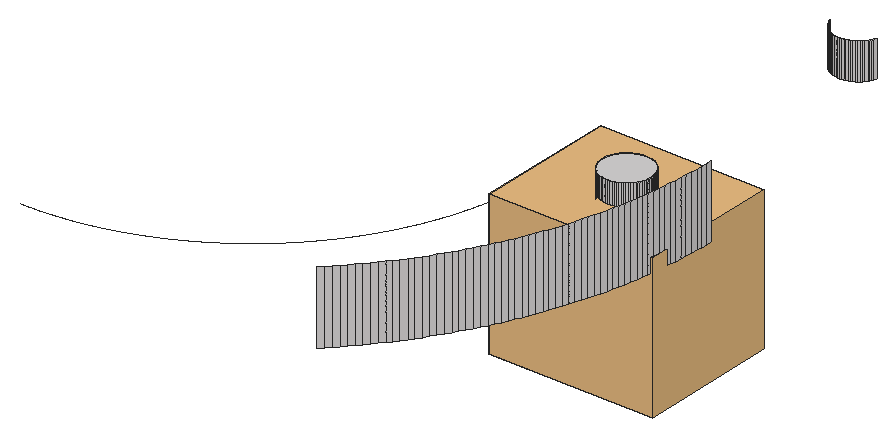
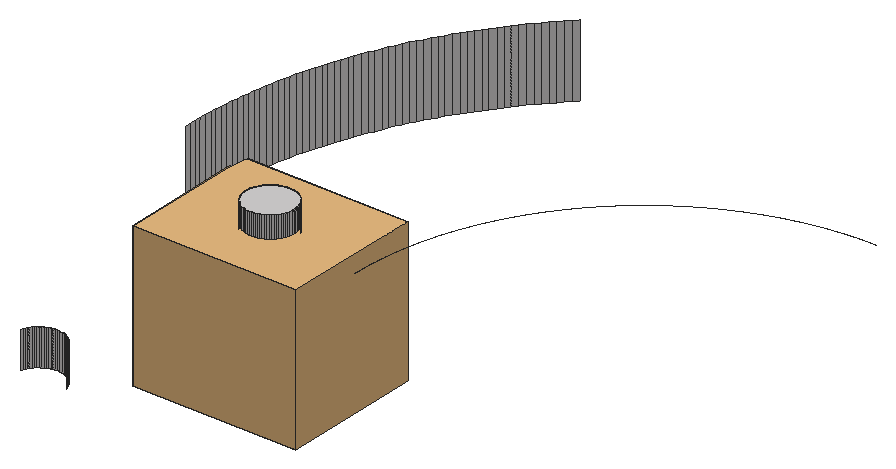
# SketchUp Ruby script. Lengths in inches.
U = 1.inch
M = Sketchup.active_model
def pt(a) = Geom::Point3d.new(a.map { |v| v * U })
def face(e, loops, mat)
  f = e.add_face(loops[0].map { |a| pt(a) })
  loops[1..].each { |l| e.add_face(l.map { |a| pt(a) }).erase! }
  f.material = f.back_material = mat if mat
  f
end
# faces: each face lists its corners as indices into pts; further lists are holes
def faces(e, pts, list, mat = nil) = list.each { |f| face(e, (f[0].is_a?(Array) ? f : [f]).map { |l| l.map { |i| pts[i] } }, mat) }
# xy, xz, yz: faces in a plane at the given z, y or x. An outline is a flat list of corners, or four numbers for a rectangle; further outlines are holes
def ring(l) = l.size == 4 ? [[l[0], l[1]], [l[2], l[1]], [l[2], l[3]], [l[0], l[3]]] : l.each_slice(2).to_a
def flat(e, list, mat, &to3) = list.each { |f| face(e, (f[0].is_a?(Array) ? f : [f]).map { |l| ring(l).map { |u, v| to3.(u, v) } }, mat) }
def xy(e, z, list, mat = nil) = flat(e, list, mat) { |x, y| [x, y, z] }
def xz(e, y, list, mat = nil) = flat(e, list, mat) { |x, z| [x, y, z] }
def yz(e, x, list, mat = nil) = flat(e, list, mat) { |y, z| [x, y, z] }
def lines(e, pts, list) = list.each { |a, b| e.add_line(pt(pts[a]), pt(pts[b])) }
# prism: a flat outline (further loops are holes) pulled along v
def prism(e, loops, v, mat = nil)
  f = face(e, loops, mat); d = Geom::Vector3d.new(v.map { |x| x * U })
  f.pushpull(f.normal.samedirection?(d) ? d.length : -d.length)
end
def box(e, o, s, mat = nil) = prism(e, [[o, [o[0] + s[0], o[1], o[2]], [o[0] + s[0], o[1] + s[1], o[2]], [o[0], o[1] + s[1], o[2]]]], [0, 0, s[2]], mat)
def at(x, y, z, deg = 0) = Geom::Transformation.translation(pt([x, y, z])) * Geom::Transformation.rotation(ORIGIN, Z_AXIS, deg.degrees)
def axes(o, x, y, z) = Geom::Transformation.new([*x, 0, *y, 0, *z, 0, *pt(o).to_a, 1])
def part(name) = M.definitions.add(name)
# library, detail: a bought-in or finely detailed component or shape, given as its bounding box
def library(name, o, s) = part(name).tap { |d| box(d.entities, o, s) }
def detail(e, o, s) = box(e.add_group.entities, o, s)
def put(e, d, t, mat = nil) = e.add_instance(d, t).tap { |i| i.material = mat if mat }
def group(e, t, mat = nil) = e.add_group.tap { |g| g.transformation = t; g.material = mat if mat }.entities
root = M.entities
M.materials.add("[Quartz Light Brown]").color = [215, 212, 212]
c1 = library("3",[-5.26,-4.28,-11.86],[13.52,11.56,11.86])
xy(root,483,[[494.91,318.7,494.59,318.74,494.44,318.78,494.29,318.83,494.15,318.89,494.01,318.96,493.875,319.05,493.75,319.14,493.63,319.24,493.52,319.36,493.42,319.48,493.33,319.6,493.25,319.74,493.18,319.88,493.12,320.02,493.07,320.17,493.04,320.33,493.01,320.48,493,320.64,493,320.8,493.02,320.95,493.04,321.11,493.08,321.26,493.13,321.41,493.19,321.55,493.26,321.69,493.35,321.83,493.44,321.95,493.54,322.07,493.65,322.18,493.77,322.28,493.9,322.37,494.04,322.45,494.18,322.52,494.32,322.58,494.47,322.63,494.625,322.67,494.78,322.6875,494.9375,322.7,495.09,322.7,495.25,322.69,495.41,322.66,495.56,322.62,495.71,322.57,495.85,322.51,495.99,322.4375,496.125,322.35,496.25,322.26,496.37,322.16,496.48,322.05,496.58,321.93,496.67,321.8,496.75,321.66,496.82,321.52,496.88,321.38,496.93,321.23,496.96,321.08,496.99,320.92,497,320.76,497,320.61,496.96,320.29,496.92,320.14,496.87,319.99,496.81,319.85,496.74,319.71,496.56,319.45,496.46,319.33,496.35,319.22,496.23,319.12,496.1,319.03,495.96,318.95,495.82,318.88,495.68,318.82,495.53,318.77,495.22,318.71,495.0625,318.7]],"[Quartz Light Brown]")
xz(root,318.7,[[494.91,480,495.0625,483]],"[Quartz Light Brown]")
xz(root,322.7,[[494.9375,480,495.09,483]],"[Quartz Light Brown]")
xz(root,342.7,[[494.91,480,495.0625,483]],"[Quartz Light Brown]")
yz(root,493,[[320.64,480,320.8,483]],"[Quartz Light Brown]")
yz(root,497,[[320.61,480,320.76,483]],"[Quartz Light Brown]")
yz(root,502,[[320.2,480,320.7,486]],"[Quartz Light Brown]")
p = [[490.87,293.83,480],[491.22,294.18,480],[491.22,294.18,486],[490.87,293.83,486],[491.5625,294.54,480],[491.5625,294.54,486],
  [491.9,294.91,480],[491.9,294.91,486],[492.24,295.27,480],[492.24,295.27,486],[492.57,295.65,480],[492.57,295.65,486],
  [492.9,296.02,480],[492.9,296.02,486],[493.22,296.4,480],[493.22,296.4,486],[493.53,296.79,480],[493.53,296.79,486],
  [493.84,297.18,480],[493.84,297.18,486],[494.15,297.57,480],[494.15,297.57,486],[494.45,297.96,480],[494.45,297.96,486],
  [494.74,298.37,480],[494.74,298.37,486],[495.03,298.77,480],[495.03,298.77,486],[495.32,299.18,480],[495.32,299.18,486],
  [495.6,299.59,480],[495.6,299.59,486],[495.87,300,480],[495.87,300,486],[496.14,300.42,480],[496.14,300.42,486],
  [496.4,300.85,480],[496.4,300.85,486],[496.66,301.27,480],[496.66,301.27,486],[496.91,301.7,480],[496.91,301.7,486],
  [497.15,302.13,480],[497.15,302.13,486],[497.4,302.57,480],[497.4,302.57,486],[497.63,303.01,480],[497.63,303.01,486],
  [497.86,303.45,480],[497.86,303.45,486],[498.08,303.89,480],[498.08,303.89,486],[498.3,304.34,480],[498.3,304.34,486],
  [498.51,304.79,480],[498.51,304.79,486],[498.71,305.25,480],[498.71,305.25,486],[498.91,305.7,480],[498.91,305.7,486],
  [499.11,306.16,480],[499.11,306.16,486],[499.29,306.62,480],[499.29,306.62,486],[499.48,307.08,480],[499.48,307.08,486],
  [499.65,307.55,480],[499.65,307.55,486],[499.82,308.02,480],[499.82,308.02,486],[499.98,308.49,480],[499.98,308.49,486],
  [500.14,308.96,480],[500.14,308.96,486],[500.29,309.43,480],[500.29,309.43,486],[500.44,309.91,480],[500.44,309.91,486],
  [500.57,310.39,480],[500.57,310.39,486],[500.71,310.87,480],[500.71,310.87,486],[500.83,311.35,480],[500.83,311.35,486],
  [500.95,311.83,480],[500.95,311.83,486],[501.0625,312.31,480],[501.0625,312.31,486],[501.17,312.8,480],[501.17,312.8,486],
  [501.27,313.29,480],[501.27,313.29,486],[501.36,313.78,480],[501.36,313.78,486],[501.45,314.27,480],[501.45,314.27,486],
  [501.53,314.76,480],[501.53,314.76,486],[501.61,315.25,480],[501.61,315.25,486],[501.67,315.74,480],[501.67,315.74,486],
  [501.74,316.23,480],[501.74,316.23,486],[501.79,316.73,480],[501.79,316.73,486],[501.84,317.22,480],[501.84,317.22,486],
  [501.88,317.72,480],[501.88,317.72,486],[501.92,318.22,480],[501.92,318.22,486],[501.95,318.71,480],[501.95,318.71,486],
  [494.59,318.74,480],[494.44,318.78,480],[494.44,318.78,483],[494.59,318.74,483],[494.75,318.72,480],[494.75,318.72,483],
  [494.91,318.7,480],[494.91,318.7,483],[495.22,318.71,480],[495.0625,318.7,480],[495.0625,318.7,483],[495.22,318.71,483],
  [495.375,318.74,480],[495.375,318.74,483],[495.53,318.77,480],[495.53,318.77,483],[501.97,319.21,480],[501.97,319.21,486],
  [494.29,318.83,480],[494.15,318.89,480],[494.15,318.89,483],[494.29,318.83,483],[495.68,318.82,480],[495.68,318.82,483],
  [495.82,318.88,480],[495.82,318.88,483],[494.01,318.96,480],[494.01,318.96,483],[495.96,318.95,480],[495.96,318.95,483],
  [496.1,319.03,480],[496.1,319.03,483],[493.875,319.05,480],[493.75,319.14,480],[493.75,319.14,483],[493.875,319.05,483],
  [496.23,319.12,480],[496.23,319.12,483],[493.63,319.24,480],[493.63,319.24,483],[496.35,319.22,480],[496.35,319.22,483],
  [493.52,319.36,480],[493.52,319.36,483],[496.46,319.33,480],[496.46,319.33,483],[501.99,319.71,480],[501.99,319.71,486],
  [496.56,319.45,480],[496.56,319.45,483],[493.42,319.48,480],[493.42,319.48,483],[493.33,319.6,480],[493.33,319.6,483],
  [496.65,319.58,480],[496.65,319.58,483],[493.25,319.74,480],[493.25,319.74,483],[496.74,319.71,480],[496.74,319.71,483],
  [493.18,319.88,480],[493.18,319.88,483],[496.81,319.85,480],[496.81,319.85,483],[502,320.2,480],[502,320.2,486],
  [496.87,319.99,480],[496.87,319.99,483],[493.12,320.02,480],[493.12,320.02,483],[493.07,320.17,480],[493.07,320.17,483],
  [496.92,320.14,480],[496.92,320.14,483],[496.96,320.29,480],[496.96,320.29,483],[493.04,320.33,480],[493.04,320.33,483],
  [493.01,320.48,480],[493.01,320.48,483],[496.98,320.45,480],[496.98,320.45,483],[497,320.61,480],[497,320.61,483],
  [493,320.64,480],[493,320.64,483],[493,320.8,480],[493.02,320.95,480],[493.02,320.95,483],[493,320.8,483],
  [496.99,320.92,480],[497,320.76,480],[497,320.76,483],[496.99,320.92,483],[496.96,321.08,480],[496.96,321.08,483],
  [493.04,321.11,480],[493.04,321.11,483],[493.08,321.26,480],[493.08,321.26,483],[496.93,321.23,480],[496.93,321.23,483],
  [496.88,321.38,480],[496.88,321.38,483],[493.13,321.41,480],[493.13,321.41,483],[493.19,321.55,480],[493.19,321.55,483],
  [496.82,321.52,480],[496.82,321.52,483],[496.75,321.66,480],[496.75,321.66,483],[493.26,321.69,480],[493.26,321.69,483],
  [493.35,321.83,480],[493.35,321.83,483],[496.67,321.8,480],[496.67,321.8,483],[493.44,321.95,480],[493.44,321.95,483],
  [496.58,321.93,480],[496.58,321.93,483],[496.48,322.05,480],[496.48,322.05,483],[493.54,322.07,480],[493.54,322.07,483],
  [496.37,322.16,480],[496.37,322.16,483],[493.65,322.18,480],[493.65,322.18,483],[493.77,322.28,480],[493.77,322.28,483],
  [496.25,322.26,480],[496.25,322.26,483],[493.9,322.37,480],[493.9,322.37,483],[496.125,322.35,480],[496.125,322.35,483],
  [494.04,322.45,480],[494.04,322.45,483],[495.85,322.51,480],[495.99,322.4375,480],[495.99,322.4375,483],[495.85,322.51,483],
  [494.18,322.52,480],[494.18,322.52,483],[494.32,322.58,480],[494.32,322.58,483],[495.71,322.57,480],[495.71,322.57,483],
  [494.47,322.63,480],[494.47,322.63,483],[494.625,322.67,480],[494.625,322.67,483],[495.41,322.66,480],[495.56,322.62,480],
  [495.56,322.62,483],[495.41,322.66,483],[494.78,322.6875,480],[494.78,322.6875,483],[494.9375,322.7,480],[494.9375,322.7,483],
  [495.09,322.7,480],[495.25,322.69,480],[495.25,322.69,483],[495.09,322.7,483],[494.59,342.74,480],[494.44,342.78,480],
  [494.44,342.78,483],[494.59,342.74,483],[494.75,342.72,480],[494.75,342.72,483],[494.91,342.7,480],[494.91,342.7,483],
  [495.22,342.71,480],[495.0625,342.7,480],[495.0625,342.7,483],[495.22,342.71,483],[495.375,342.74,480],[495.375,342.74,483],
  [495.53,342.77,480],[495.53,342.77,483],[494.29,342.83,480],[494.15,342.89,480],[494.15,342.89,483],[494.29,342.83,483],
  [495.68,342.82,480],[495.68,342.82,483],[495.82,342.88,480],[495.82,342.88,483],[494.01,342.96,480],[494.01,342.96,483],
  [495.96,342.95,480],[495.96,342.95,483],[496.1,343.03,480],[496.1,343.03,483],[493.875,343.05,480],[493.75,343.14,480],
  [493.75,343.14,483],[493.875,343.05,483],[496.23,343.12,480],[496.23,343.12,483],[493.63,343.24,480],[493.63,343.24,483],
  [496.35,343.22,480],[496.35,343.22,483],[493.52,343.36,480],[493.52,343.36,483],[496.46,343.33,480],[496.46,343.33,483],
  [496.56,343.45,480],[496.56,343.45,483],[493.42,343.48,480],[493.42,343.48,483],[493.33,343.6,480],[493.33,343.6,483],
  [496.65,343.58,480],[496.65,343.58,483],[493.25,343.74,480],[493.25,343.74,483],[496.74,343.71,480],[496.74,343.71,483],
  [493.18,343.88,480],[493.18,343.88,483],[496.81,343.85,480],[496.81,343.85,483],[496.87,343.99,480],[496.87,343.99,483],
  [493.12,344.02,480],[493.12,344.02,483],[493.07,344.17,480],[493.07,344.17,483],[496.92,344.14,480],[496.92,344.14,483],
  [464,296.7,480],[464.3125,296.7,480],[464.63,296.71,480],[464.94,296.72,480],[465.26,296.73,480],[465.57,296.75,480],
  [465.88,296.77,480],[466.2,296.8,480],[466.51,296.83,480],[466.82,296.87,480],[467.13,296.91,480],[467.44,296.95,480],
  [467.75,297,480],[468.0625,297.05,480],[468.375,297.1,480],[468.68,297.16,480],[468.99,297.23,480],[469.3,297.29,480],
  [469.6,297.36,480],[469.91,297.4375,480],[470.21,297.52,480],[470.51,297.6,480],[470.82,297.6875,480],[471.12,297.78,480],
  [471.42,297.875,480],[471.71,297.97,480],[472.01,298.08,480],[472.31,298.18,480],[472.6,298.3,480],[472.89,298.41,480],
  [473.18,298.53,480],[473.47,298.65,480],[473.76,298.78,480],[474.05,298.91,480],[474.33,299.04,480],[474.61,299.18,480],
  [474.9,299.32,480],[475.17,299.46,480],[475.45,299.61,480],[475.73,299.76,480],[476,299.92,480],[476.27,300.08,480],
  [476.54,300.24,480],[476.81,300.4,480],[477.07,300.57,480],[477.33,300.75,480],[477.59,300.92,480],[477.85,301.1,480],
  [478.11,301.28,480],[478.36,301.47,480],[478.61,301.66,480],[478.86,301.85,480],[479.1,302.05,480],[479.35,302.25,480],
  [479.59,302.45,480],[479.82,302.66,480],[480.06,302.87,480],[480.29,303.08,480],[480.52,303.29,480],[480.75,303.51,480],
  [480.97,303.73,480],[481.19,303.95,480],[481.41,304.18,480],[481.625,304.41,480],[481.84,304.64,480],[482.04,304.875,480],
  [482.25,305.11,480],[482.45,305.35,480],[482.65,305.6,480],[482.85,305.84,480],[483.04,306.09,480],[483.23,306.34,480],
  [483.42,306.59,480],[483.6,306.85,480],[483.78,307.11,480],[483.96,307.37,480],[484.13,307.63,480],[484.3,307.89,480],
  [484.46,308.16,480],[484.625,308.43,480],[484.78,308.7,480],[484.94,308.97,480],[485.09,309.25,480],[485.24,309.53,480],
  [485.38,309.81,480],[485.52,310.09,480],[485.66,310.37,480],[485.8,310.65,480],[485.93,310.9375,480],[486.05,311.23,480],
  [486.17,311.52,480],[486.29,311.81,480],[486.41,312.1,480],[486.52,312.39,480],[486.625,312.69,480],[486.73,312.99,480],
  [486.83,313.28,480],[486.92,313.58,480],[487.01,313.88,480],[487.1,314.1875,480],[487.18,314.49,480],[487.26,314.79,480],
  [487.34,315.1,480],[487.41,315.4,480],[487.48,315.71,480],[487.54,316.02,480],[487.6,316.33,480],[487.65,316.64,480],
  [487.7,316.95,480],[487.75,317.26,480],[487.79,317.57,480],[487.83,317.88,480],[487.87,318.19,480],[487.9,318.5,480],
  [487.93,318.82,480],[487.95,319.13,480],[487.97,319.44,480],[487.98,319.76,480],[487.99,320.07,480],[488,320.39,480],
  [488,320.7,480]]
faces(root,p,[[0,1,2,3],[1,4,5,2],[4,6,7,5],[6,8,9,7],[8,10,11,9],[10,12,13,11],[12,14,15,13],[14,16,17,15],
  [16,18,19,17],[18,20,21,19],[20,22,23,21],[22,24,25,23],[24,26,27,25],[26,28,29,27],[28,30,31,29],[30,32,33,31],
  [32,34,35,33],[34,36,37,35],[36,38,39,37],[38,40,41,39],[40,42,43,41],[42,44,45,43],[44,46,47,45],[46,48,49,47],
  [48,50,51,49],[50,52,53,51],[52,54,55,53],[54,56,57,55],[56,58,59,57],[58,60,61,59],[60,62,63,61],[62,64,65,63],
  [64,66,67,65],[66,68,69,67],[68,70,71,69],[70,72,73,71],[72,74,75,73],[74,76,77,75],[76,78,79,77],[78,80,81,79],
  [80,82,83,81],[82,84,85,83],[84,86,87,85],[86,88,89,87],[88,90,91,89],[90,92,93,91],[92,94,95,93],[94,96,97,95],
  [96,98,99,97],[98,100,101,99],[100,102,103,101],[102,104,105,103],[104,106,107,105],[106,108,109,107],[108,110,111,109],[110,112,113,111],
  [114,115,116,117],[118,114,117,119],[120,118,119,121],[122,123,124,125],[126,122,125,127],[128,126,127,129],[112,130,131,113],[132,133,134,135],
  [115,132,135,116],[136,128,129,137],[138,136,137,139],[133,140,141,134],[142,138,139,143],[144,142,143,145],[146,147,148,149],[140,146,149,141],
  [150,144,145,151],[147,152,153,148],[154,150,151,155],[152,156,157,153],[158,154,155,159],[130,160,161,131],[162,158,159,163],[156,164,165,157],
  [164,166,167,165],[168,162,163,169],[166,170,171,167],[172,168,169,173],[170,174,175,171],[176,172,173,177],[160,178,179,161],[180,176,177,181],
  [174,182,183,175],[182,184,185,183],[186,180,181,187],[188,186,187,189],[184,190,191,185],[190,192,193,191],[194,188,189,195],[196,194,195,197],
  [192,198,199,193],[200,201,202,203],[204,205,206,207],[208,204,207,209],[201,210,211,202],[210,212,213,211],[214,208,209,215],[216,214,215,217],
  [212,218,219,213],[218,220,221,219],[222,216,217,223],[224,222,223,225],[220,226,227,221],[226,228,229,227],[230,224,225,231],[228,232,233,229],
  [234,230,231,235],[236,234,235,237],[232,238,239,233],[240,236,237,241],[238,242,243,239],[242,244,245,243],[246,240,241,247],[244,248,249,245],
  [250,246,247,251],[248,252,253,249],[254,255,256,257],[255,250,251,256],[252,258,259,253],[258,260,261,259],[262,254,257,263],[260,264,265,261],
  [264,266,267,265],[268,269,270,271],[269,262,263,270],[266,272,273,267],[272,274,275,273],[276,277,278,279],[277,268,271,278],[280,281,282,283],
  [284,280,283,285],[286,284,285,287],[288,289,290,291],[292,288,291,293],[294,292,293,295],[296,297,298,299],[281,296,299,282],[300,294,295,301],
  [302,300,301,303],[297,304,305,298],[306,302,303,307],[308,306,307,309],[310,311,312,313],[304,310,313,305],[314,308,309,315],[311,316,317,312],
  [318,314,315,319],[316,320,321,317],[322,318,319,323],[324,322,323,325],[320,326,327,321],[326,328,329,327],[330,324,325,331],[328,332,333,329],
  [334,330,331,335],[332,336,337,333],[338,334,335,339],[340,338,339,341],[336,342,343,337],[342,344,345,343],[346,340,341,347]],"[Quartz Light Brown]")
lines(root,p,[[348,349],[349,350],[350,351],[351,352],[352,353],[353,354],[354,355],[355,356],[356,357],[357,358],[358,359],[359,360],
  [360,361],[361,362],[362,363],[363,364],[364,365],[365,366],[366,367],[367,368],[368,369],[369,370],[370,371],[371,372],
  [372,373],[373,374],[374,375],[375,376],[376,377],[377,378],[378,379],[379,380],[380,381],[381,382],[382,383],[383,384],
  [384,385],[385,386],[386,387],[387,388],[388,389],[389,390],[390,391],[391,392],[392,393],[393,394],[394,395],[395,396],
  [396,397],[397,398],[398,399],[399,400],[400,401],[401,402],[402,403],[403,404],[404,405],[405,406],[406,407],[407,408],
  [408,409],[409,410],[410,411],[411,412],[412,413],[413,414],[414,415],[415,416],[416,417],[417,418],[418,419],[419,420],
  [420,421],[421,422],[422,423],[423,424],[424,425],[425,426],[426,427],[427,428],[428,429],[429,430],[430,431],[431,432],
  [432,433],[433,434],[434,435],[435,436],[436,437],[437,438],[438,439],[439,440],[440,441],[441,442],[442,443],[443,444],
  [444,445],[445,446],[446,447],[447,448],[448,449],[449,450],[450,451],[451,452],[452,453],[453,454],[454,455],[455,456],
  [456,457],[457,458],[458,459],[459,460],[460,461],[461,462],[462,463],[463,464],[464,465],[465,466],[466,467],[467,468]])
put(root,c1,axes([496.5,319.2,481.25],[-1,0,0],[0,1,0],[0,0,1]),"[Quartz Light Brown]")
